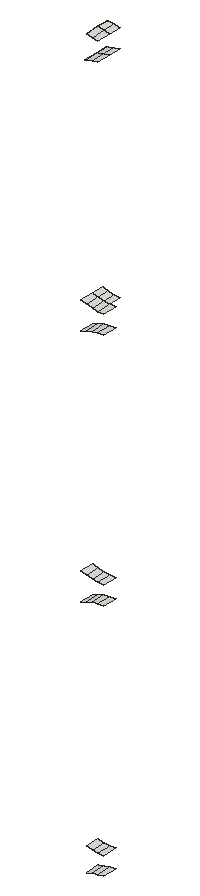
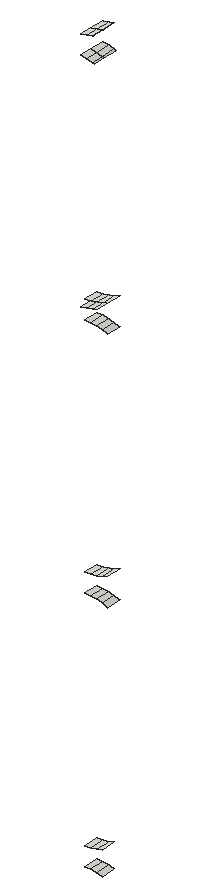
# SketchUp Ruby script. Lengths in inches.
U = 1.inch
M = Sketchup.active_model
def pt(a) = Geom::Point3d.new(a.map { |v| v * U })
def face(e, loops, mat)
  f = e.add_face(loops[0].map { |a| pt(a) })
  loops[1..].each { |l| e.add_face(l.map { |a| pt(a) }).erase! }
  f.material = f.back_material = mat if mat
  f
end
# faces: each face lists its corners as indices into pts; further lists are holes
def faces(e, pts, list, mat = nil) = list.each { |f| face(e, (f[0].is_a?(Array) ? f : [f]).map { |l| l.map { |i| pts[i] } }, mat) }
# xy, xz, yz: faces in a plane at the given z, y or x. An outline is a flat list of corners, or four numbers for a rectangle; further outlines are holes
def ring(l) = l.size == 4 ? [[l[0], l[1]], [l[2], l[1]], [l[2], l[3]], [l[0], l[3]]] : l.each_slice(2).to_a
def flat(e, list, mat, &to3) = list.each { |f| face(e, (f[0].is_a?(Array) ? f : [f]).map { |l| ring(l).map { |u, v| to3.(u, v) } }, mat) }
def xy(e, z, list, mat = nil) = flat(e, list, mat) { |x, y| [x, y, z] }
def xz(e, y, list, mat = nil) = flat(e, list, mat) { |x, z| [x, y, z] }
def yz(e, x, list, mat = nil) = flat(e, list, mat) { |y, z| [x, y, z] }
def lines(e, pts, list) = list.each { |a, b| e.add_line(pt(pts[a]), pt(pts[b])) }
# prism: a flat outline (further loops are holes) pulled along v
def prism(e, loops, v, mat = nil)
  f = face(e, loops, mat); d = Geom::Vector3d.new(v.map { |x| x * U })
  f.pushpull(f.normal.samedirection?(d) ? d.length : -d.length)
end
def box(e, o, s, mat = nil) = prism(e, [[o, [o[0] + s[0], o[1], o[2]], [o[0] + s[0], o[1] + s[1], o[2]], [o[0], o[1] + s[1], o[2]]]], [0, 0, s[2]], mat)
def at(x, y, z, deg = 0) = Geom::Transformation.translation(pt([x, y, z])) * Geom::Transformation.rotation(ORIGIN, Z_AXIS, deg.degrees)
def axes(o, x, y, z) = Geom::Transformation.new([*x, 0, *y, 0, *z, 0, *pt(o).to_a, 1])
def part(name) = M.definitions.add(name)
# library, detail: a bought-in or finely detailed component or shape, given as its bounding box
def library(name, o, s) = part(name).tap { |d| box(d.entities, o, s) }
def detail(e, o, s) = box(e.add_group.entities, o, s)
def put(e, d, t, mat = nil) = e.add_instance(d, t).tap { |i| i.material = mat if mat }
def group(e, t, mat = nil) = e.add_group.tap { |g| g.transformation = t; g.material = mat if mat }.entities
root = M.entities
p = [[81.558,138.787,9.861],[81.867,138.787,9.938],[81.867,138,9.938],[81.558,138,9.861],[82.182,138.787,9.984],[82.182,138,9.984],
  [82.5,138.787,10],[82.5,138,10],[82.182,138.787,11.016],[81.867,138.787,11.062],[81.867,138,11.062],[82.182,138,11.016],
  [82.5,138.787,11],[82.5,138,11],[81.558,138.787,11.139],[81.558,138,11.139],[81.258,138.787,22.753],[81.558,138.787,22.861],
  [81.558,138,22.861],[81.258,138,22.753],[81.867,138.787,22.938],[81.867,138,22.938],[82.182,138.787,22.984],[82.182,138,22.984],
  [82.5,138.787,23],[82.5,138,23],[82.182,138.787,24.016],[81.867,138.787,24.062],[81.867,138,24.062],[82.182,138,24.016],
  [82.5,138.787,24],[82.5,138,24],[81.558,138.787,24.139],[81.258,138.787,24.247],[81.258,138,24.247],[81.558,138,24.139],
  [81.258,138.787,35.753],[81.558,138.787,35.861],[81.558,138,35.861],[81.258,138,35.753],[81.867,138.787,35.938],[81.867,138,35.938],
  [82.182,138.787,35.984],[82.182,138,35.984],[82.5,138.787,36],[82.5,138,36],[82.182,138.787,37.016],[81.867,138.787,37.062],
  [81.867,138,37.062],[82.182,138,37.016],[82.5,138.787,37],[82.5,138,37],[81.867,139.4375,37.062],[82.182,139.4375,37.016],
  [81.558,138.787,37.139],[81.258,138.787,37.247],[81.258,138,37.247],[81.558,138,37.139],[81.258,139.4375,37.247],[81.558,139.4375,37.139],
  [81.558,138,48.861],[81.457,138,48.824],[81.457,138.787,48.824],[81.558,138.787,48.861],[81.558,139.4375,48.861],[81.457,139.4375,48.824],
  [81.867,138.787,48.938],[81.867,138,48.938],[82.182,138.787,48.984],[82.182,138,48.984],[81.867,139.4375,48.938],[82.182,139.4375,48.984],
  [82.182,138.787,50.016],[81.867,138.787,50.062],[81.867,138,50.062],[82.182,138,50.016],[81.867,139.4375,50.062],[82.182,139.4375,50.016],
  [81.558,138.787,50.139],[81.557,138.787,50.14],[81.557,138,50.14],[81.558,138,50.139],[81.557,139.4375,50.14],[81.558,139.4375,50.139]]
faces(root,p,[[0,1,2,3],[1,4,5,2],[4,6,7,5],[8,9,10,11],[12,8,11,13],[9,14,15,10],[16,17,18,19],[17,20,21,18],
  [20,22,23,21],[22,24,25,23],[26,27,28,29],[30,26,29,31],[32,33,34,35],[27,32,35,28],[36,37,38,39],[37,40,41,38],
  [40,42,43,41],[42,44,45,43],[46,47,48,49],[50,46,49,51],[52,47,46,53],[54,55,56,57],[47,54,57,48],[58,55,54,59],
  [59,54,47,52],[60,61,62,63],[64,63,62,65],[63,66,67,60],[66,68,69,67],[70,66,63,64],[71,68,66,70],[72,73,74,75],
  [76,73,72,77],[78,79,80,81],[73,78,81,74],[82,79,78,83],[83,78,73,76]])
